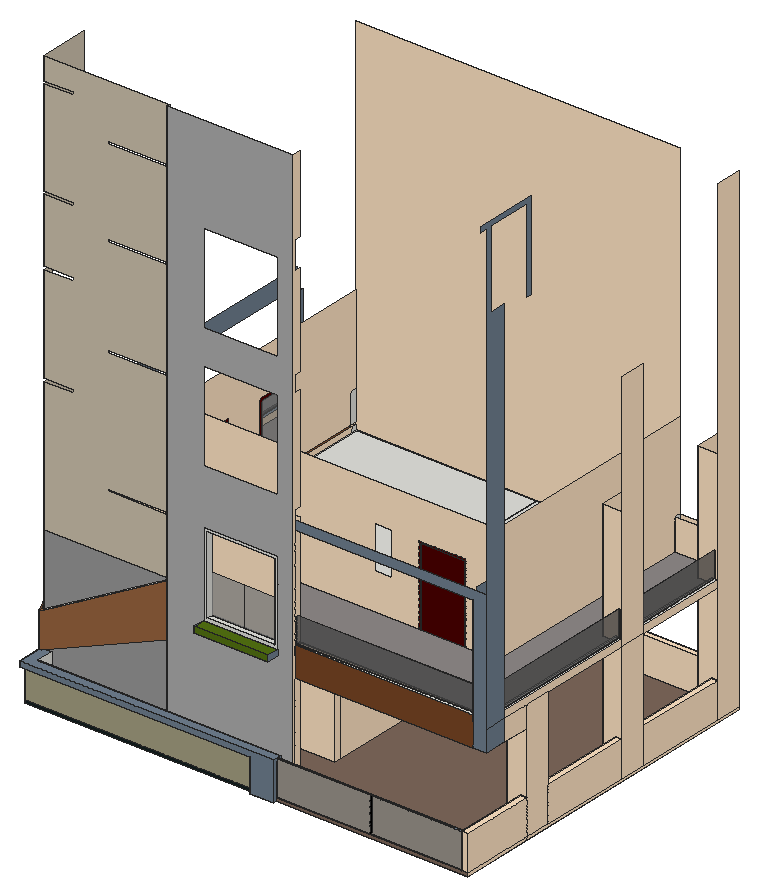
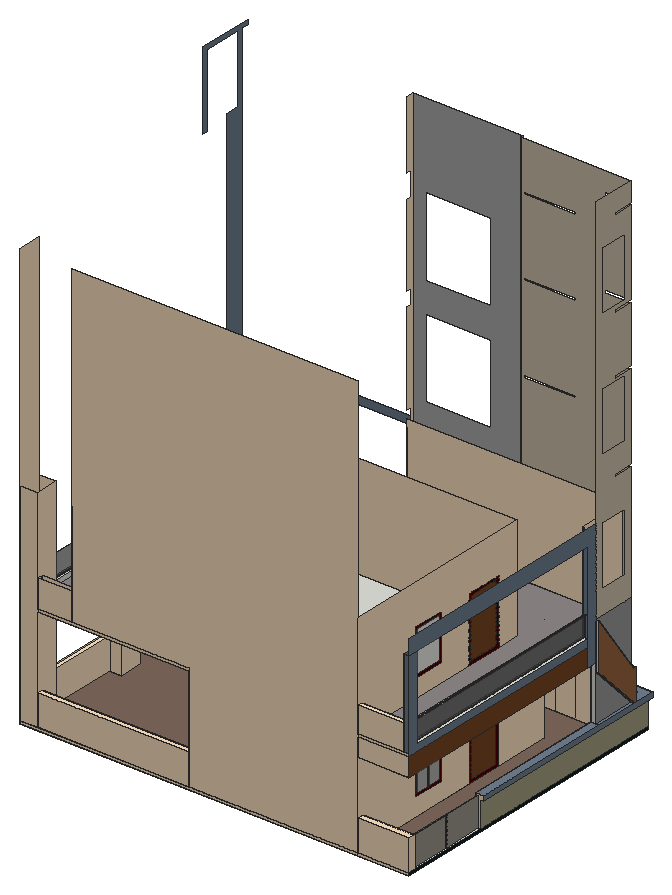
# SketchUp Ruby script. Lengths in inches.
U = 1.inch
M = Sketchup.active_model
def pt(a) = Geom::Point3d.new(a.map { |v| v * U })
def face(e, loops, mat)
  f = e.add_face(loops[0].map { |a| pt(a) })
  loops[1..].each { |l| e.add_face(l.map { |a| pt(a) }).erase! }
  f.material = f.back_material = mat if mat
  f
end
# faces: each face lists its corners as indices into pts; further lists are holes
def faces(e, pts, list, mat = nil) = list.each { |f| face(e, (f[0].is_a?(Array) ? f : [f]).map { |l| l.map { |i| pts[i] } }, mat) }
# xy, xz, yz: faces in a plane at the given z, y or x. An outline is a flat list of corners, or four numbers for a rectangle; further outlines are holes
def ring(l) = l.size == 4 ? [[l[0], l[1]], [l[2], l[1]], [l[2], l[3]], [l[0], l[3]]] : l.each_slice(2).to_a
def flat(e, list, mat, &to3) = list.each { |f| face(e, (f[0].is_a?(Array) ? f : [f]).map { |l| ring(l).map { |u, v| to3.(u, v) } }, mat) }
def xy(e, z, list, mat = nil) = flat(e, list, mat) { |x, y| [x, y, z] }
def xz(e, y, list, mat = nil) = flat(e, list, mat) { |x, z| [x, y, z] }
def yz(e, x, list, mat = nil) = flat(e, list, mat) { |y, z| [x, y, z] }
def lines(e, pts, list) = list.each { |a, b| e.add_line(pt(pts[a]), pt(pts[b])) }
# prism: a flat outline (further loops are holes) pulled along v
def prism(e, loops, v, mat = nil)
  f = face(e, loops, mat); d = Geom::Vector3d.new(v.map { |x| x * U })
  f.pushpull(f.normal.samedirection?(d) ? d.length : -d.length)
end
def box(e, o, s, mat = nil) = prism(e, [[o, [o[0] + s[0], o[1], o[2]], [o[0] + s[0], o[1] + s[1], o[2]], [o[0], o[1] + s[1], o[2]]]], [0, 0, s[2]], mat)
def at(x, y, z, deg = 0) = Geom::Transformation.translation(pt([x, y, z])) * Geom::Transformation.rotation(ORIGIN, Z_AXIS, deg.degrees)
def axes(o, x, y, z) = Geom::Transformation.new([*x, 0, *y, 0, *z, 0, *pt(o).to_a, 1])
def part(name) = M.definitions.add(name)
# library, detail: a bought-in or finely detailed component or shape, given as its bounding box
def library(name, o, s) = part(name).tap { |d| box(d.entities, o, s) }
def detail(e, o, s) = box(e.add_group.entities, o, s)
def put(e, d, t, mat = nil) = e.add_instance(d, t).tap { |i| i.material = mat if mat }
def group(e, t, mat = nil) = e.add_group.tap { |g| g.transformation = t; g.material = mat if mat }.entities
root = M.entities
M.materials.add("[0008_LavenderBlush]").color = [255, 240, 245]
M.materials.add("[0012_Bisque]").color = [255, 228, 196]
M.materials.add("[0021_DarkRed]").color = [76, 0, 0]
M.materials.add("[0021_DarkRed]1").color = [81, 0, 0]
M.materials.add("[0078_DarkSlateGray]").color = [19, 33, 33]
M.materials.add("[0111_SlateGray]").color = [112, 128, 144]
M.materials.add("[0136_Charcoal]").color = [35, 35, 35]
M.materials.add("[0137_Black]").color = [0, 0, 0]
M.materials.add("[Beadboard]").color = [153, 100, 63]
M.materials.add("[Carrera Marble]").color = [153, 153, 153]
M.materials.add("[Cladding Siding White]").color = [173, 173, 173]
M.materials.add("[Granite Brown]").color = [126, 104, 91]
M.materials.add("[Siding Rusty Metal]").color = [206, 195, 174]
M.materials.add("[Stone Coursed Rough]").color = [165, 160, 130]
M.materials.add("[Stone Marble]").color = [143, 138, 136]
M.materials.add("[Stone Masonry Multi]").color = [155, 149, 140]
M.materials.add("[Translucent Glass Gray]").color = [84, 84, 84]
M.materials["[Translucent Glass Gray]"].alpha = 0.5
M.materials.add("[Translucent Glass Gray]1").color = [128, 128, 128]
M.materials["[Translucent Glass Gray]1"].alpha = 0.5
M.materials.add("[Translucent Resin Crush Gray]").color = [153, 153, 153]
M.materials["[Translucent Resin Crush Gray]"].alpha = 0.8
M.materials.add("[Vegetation Blur 03]").color = [83, 114, 18]
M.materials.add("[Wood Veneer 01]").color = [120, 70, 37]
xy(root,0,[[948,0,948,12,24,12,24,1392,1824,1392,1824,12,1044,12,1044,0]])
xy(root,12,[[1044,12,1800,19.07],[1800,12,1824,312],[1044,19.07,1800,28.21],[1044,28.21,1800,36],[534,96,1044,108],
  [24,108,1044,132],[24,132,48,312],[24,312,48,978],[264,312,264,1392,1044,1392,1044,1368,288,1368,288,336,1044,336,1044,312],[1745,312,1824,420],
  [288,336,1020,1368],[1020,336,1044,1368],[1800,420,1824,798],[1745,798,1824,906],[1800,906,1824,1284],
  [24,978,36,1362],[36,978,41.76,1362],[41.76,978,48,1362],[1745,1284,1824,1392],[24,1362,264,1392],
  [1044,1368,1745,1392]])
xy(root,12,[[54,36,1800,36,1800,312,1745,312,1745,420,1800,420,1800,798,1745,798,1745,906,1800,906,1800,1284,1745,1284,1745,1368,1044,1368,1044,312,264,312,264,1362,48,1362,48,132,1044,132,1044,96,534,96,534,108,54,108]],"[Granite Brown]")
xy(root,19,[[1032,778.41,1044,981.6]],"[Wood Veneer 01]")
xy(root,132,[[12,0,12,978,24,978,24,12,948,12,948,0]],"[0111_SlateGray]")
xy(root,142.6875,[[1032,490.33,1044,626.21],[1032,1100.27,1044,1236.15]],"[Wood Veneer 01]")
xy(root,144.9375,[[36,978,41.76,1362]],"[Stone Masonry Multi]")
xy(root,151.1875,[[1044,19.07,1800,28.21]],"[0111_SlateGray]")
xy(root,156,[[1800,12,1824,312],[1800,420,1824,798],[1800,906,1824,1284],[24,1362,264,1392],[1044,1368,1745,1392]],"[0012_Bisque]")
xy(root,156,[[12,0,1044,0,1044,36,54,36,54,108,24,108,24,96,12,96],[12,108,24,312],[12,312,48,978]],"[0111_SlateGray]")
xy(root,156,[[12,96,24,108]],"[Beadboard]")
xy(root,300,[[12,96,24,108]],"[Beadboard]")
xy(root,335.4375,[[1032,490.33,1044,626.21],[1032,778.41,1044,981.6],[1032,1100.27,1044,1236.15]],"[Wood Veneer 01]")
xy(root,408,[[1800,132,1824,312]],"[0012_Bisque]")
xy(root,408,[[1044,108,1824,132],[24,312,24,1392,264,1392,264,1374,42,1374,42,312]],"[Wood Veneer 01]")
xy(root,471.68,[[683.08,48,983.45,96]],"[0111_SlateGray]")
xy(root,492,[[1800,132,1824,312],[288,336,1020,1368],[1020,336,1044,1368]])
xy(root,492,[[1298.29,369.5625,1292.07,370.38,1286.29,372.78,1281.32,376.59,1277.5,381.5625,1275.1,387.35,1274.29,393.5625,1275.1,399.77,1277.5,405.5625,1281.32,410.53,1286.29,414.35,1292.07,416.74,1298.29,417.5625,1304.5,416.74,1310.29,414.35,1315.26,410.53,1319.07,405.5625,1321.47,399.77,1322.29,393.5625,1321.47,387.35,1319.07,381.5625,1315.26,376.59,1310.29,372.78,1304.5,370.38],[1588.47,369.5625,1582.26,370.38,1576.47,372.78,1571.5,376.59,1567.6875,381.5625,1565.29,387.35,1564.47,393.5625,1565.29,399.77,1567.6875,405.5625,1571.5,410.53,1576.47,414.35,1582.26,416.74,1588.47,417.5625,1594.69,416.74,1600.47,414.35,1605.44,410.53,1609.26,405.5625,1611.66,399.77,1612.47,393.5625,1611.66,387.35,1609.26,381.5625,1605.44,376.59,1600.47,372.78,1594.69,370.38],[1588.47,625.0625,1582.26,625.88,1576.47,628.28,1571.5,632.09,1567.6875,637.0625,1565.29,642.85,1564.47,649.0625,1565.29,655.27,1567.6875,661.0625,1571.5,666.03,1576.47,669.85,1582.26,672.24,1588.47,673.0625,1594.69,672.24,1600.47,669.85,1605.44,666.03,1609.26,661.0625,1611.66,655.27,1612.47,649.0625,1611.66,642.85,1609.26,637.0625,1605.44,632.09,1600.47,628.28,1594.69,625.88],[1298.29,648.9375,1292.07,649.76,1286.29,652.15,1281.32,655.97,1277.5,660.9375,1275.1,666.73,1274.29,672.9375,1275.1,679.15,1277.5,684.9375,1281.32,689.91,1286.29,693.72,1292.07,696.12,1298.29,696.9375,1304.5,696.12,1310.29,693.72,1315.26,689.91,1319.07,684.9375,1321.47,679.15,1322.29,672.9375,1321.47,666.73,1319.07,660.9375,1315.26,655.97,1310.29,652.15,1304.5,649.76],[1588.47,1073.625,1582.26,1074.44,1576.47,1076.84,1571.5,1080.65,1567.6875,1085.625,1565.29,1091.41,1564.47,1097.625,1565.29,1103.84,1567.6875,1109.625,1571.5,1114.6,1576.47,1118.41,1582.26,1120.81,1588.47,1121.625,1594.69,1120.81,1600.47,1118.41,1605.44,1114.6,1609.26,1109.625,1611.66,1103.84,1612.47,1097.625,1611.66,1091.41,1609.26,1085.625,1605.44,1080.65,1600.47,1076.84,1594.69,1074.44],
  [1298.29,1135.0625,1292.07,1135.88,1286.29,1138.28,1281.32,1142.09,1277.5,1147.0625,1275.1,1152.85,1274.29,1159.0625,1275.1,1165.27,1277.5,1171.0625,1281.32,1176.03,1286.29,1179.85,1292.07,1182.24,1298.29,1183.0625,1304.5,1182.24,1310.29,1179.85,1315.26,1176.03,1319.07,1171.0625,1321.47,1165.27,1322.29,1159.0625,1321.47,1152.85,1319.07,1147.0625,1315.26,1142.09,1310.29,1138.28,1304.5,1135.88]],"[0008_LavenderBlush]")
xy(root,492,[[[48,132,48,312,1044,312,1044,1392,1745,1392,1745,1284,1824,1284,1824,906,1745,906,1745,798,1824,798,1824,420,1745,420,1745,312,1800,312,1800,132],[1588.47,1073.625,1594.69,1074.44,1600.47,1076.84,1605.44,1080.65,1609.26,1085.625,1611.66,1091.41,1612.47,1097.625,1611.66,1103.84,1609.26,1109.625,1605.44,1114.6,1600.47,1118.41,1594.69,1120.81,1588.47,1121.625,1582.26,1120.81,1576.47,1118.41,1571.5,1114.6,1567.6875,1109.625,1565.29,1103.84,1564.47,1097.625,1565.29,1091.41,1567.6875,1085.625,1571.5,1080.65,1576.47,1076.84,1582.26,1074.44],[1588.47,625.0625,1594.69,625.88,1600.47,628.28,1605.44,632.09,1609.26,637.0625,1611.66,642.85,1612.47,649.0625,1611.66,655.27,1609.26,661.0625,1605.44,666.03,1600.47,669.85,1594.69,672.24,1588.47,673.0625,1582.26,672.24,1576.47,669.85,1571.5,666.03,1567.6875,661.0625,1565.29,655.27,1564.47,649.0625,1565.29,642.85,1567.6875,637.0625,1571.5,632.09,1576.47,628.28,1582.26,625.88],[1588.47,369.5625,1594.69,370.38,1600.47,372.78,1605.44,376.59,1609.26,381.5625,1611.66,387.35,1612.47,393.5625,1611.66,399.77,1609.26,405.5625,1605.44,410.53,1600.47,414.35,1594.69,416.74,1588.47,417.5625,1582.26,416.74,1576.47,414.35,1571.5,410.53,1567.6875,405.5625,1565.29,399.77,1564.47,393.5625,1565.29,387.35,1567.6875,381.5625,1571.5,376.59,1576.47,372.78,1582.26,370.38],[1298.29,369.5625,1304.5,370.38,1310.29,372.78,1315.26,376.59,1319.07,381.5625,1321.47,387.35,1322.29,393.5625,1321.47,399.77,1319.07,405.5625,1315.26,410.53,1310.29,414.35,1304.5,416.74,1298.29,417.5625,1292.07,416.74,1286.29,414.35,1281.32,410.53,1277.5,405.5625,1275.1,399.77,1274.29,393.5625,1275.1,387.35,1277.5,381.5625,1281.32,376.59,1286.29,372.78,1292.07,370.38],[1298.29,648.9375,1304.5,649.76,1310.29,652.15,1315.26,655.97,1319.07,660.9375,1321.47,666.73,1322.29,672.9375,1321.47,679.15,1319.07,684.9375,1315.26,689.91,1310.29,693.72,1304.5,696.12,1298.29,696.9375,1292.07,696.12,1286.29,693.72,1281.32,689.91,1277.5,684.9375,1275.1,679.15,1274.29,672.9375,1275.1,666.73,1277.5,660.9375,1281.32,655.97,1286.29,652.15,1292.07,649.76],[1298.29,1135.0625,1304.5,1135.88,1310.29,1138.28,1315.26,1142.09,1319.07,1147.0625,1321.47,1152.85,1322.29,1159.0625,1321.47,1165.27,1319.07,1171.0625,1315.26,1176.03,1310.29,1179.85,1304.5,1182.24,1298.29,1183.0625,1292.07,1182.24,1286.29,1179.85,1281.32,1176.03,1277.5,1171.0625,1275.1,1165.27,1274.29,1159.0625,1275.1,1152.85,1277.5,1147.0625,1281.32,1142.09,1286.29,1138.28,1292.07,1135.88]],[42,312,264,1374]],"[Wood Veneer 01]")
xy(root,495.68,[[683.08,48,983.45,96]],"[Vegetation Blur 03]")
xy(root,504,[[48,1368,264,1392],[1584,1368,1745,1392]])
xy(root,504,[[48,132,1767.4375,132,1767.4375,199.52,1800,199.52,1800,798,1745,798,1745,906,1800,906,1800,1284,1745,1284,1745,1368,1584,1368,1584,468,1446.53,468,1446.53,469.5,1268.41,469.5,1268.41,468,264,468,264,1368,48,1368]],"[Stone Marble]")
xy(root,507.68,[[695.08,96,971.45,120]])
xy(root,522,[[1800,199.52,1812,798],[1812,199.52,1813.5,798],[1813.5,199.52,1824,798],[1800,906,1812,1284],[1812,906,1813.5,1284],
  [1813.5,906,1824,1284]])
xy(root,528,[[1044,108,1767.4375,118.5],[1044,118.5,1767.4375,120],[24,360,35,1350],[35,360,36,1350]])
xy(root,528,[[1044,120,1767.4375,132]],"[0012_Bisque]")
xy(root,528,[[36,360,48,1350]],"[0111_SlateGray]")
xy(root,621,[[35,360,36,1350]])
xy(root,624,[[48,1368,264,1392]],"[0012_Bisque]")
xz(root,0,[[948,0,1044,0,1044,156,12,156,12,132,948,132]],"[0111_SlateGray]")
xz(root,12,[[1800,12,1824,156]],"[0012_Bisque]")
xz(root,12,[[24,0,948,12]],"[0078_DarkSlateGray]")
xz(root,12,[[1044,0,1824,12]],"[Granite Brown]")
xz(root,12,[[24,12,948,132]],"[Stone Coursed Rough]")
xz(root,19.07,[[1422,12,1429.54,151.1875]],"[0137_Black]")
xz(root,19.07,[[1044,12,1422,151.1875],[1429.54,12,1800,151.1875]],"[Stone Masonry Multi]")
xz(root,28.21,[[1044,12,1800,151.1875]],"[Stone Masonry Multi]")
xz(root,36,[[54,12,1044,156]])
xz(root,48,[[683.08,471.68,983.45,495.68]],"[Vegetation Blur 03]")
xz(root,96,[[683.08,471.68,983.45,495.68],[[683.08,495.68,983.45,837.43],[695.08,507.68,971.45,825.43]]])
xz(root,96,[[12,156,24,156,534,373.64,534,588,24,300,12,300]],"[Beadboard]")
xz(root,96,[[[534,12,1044,2319.6],[683.08,471.68,983.45,837.43],[683.08,1057.8,983.45,1423.55],[683.08,1562.74,983.45,1928.49]]],"[Cladding Siding White]")
xz(root,108,[[24,156,24,300,534,588,534,373.64]])
xz(root,108,[[1767.4375,408,1824,408,1824,984,1044,984,1044,948,1767.4375,948]],"[0111_SlateGray]")
xz(root,108,[[54,12,534,12,534,373.64,24,156,54,156],[24,300,534,588,24,588]],"[Carrera Marble]")
xz(root,108,[[[24,588,534,588,534,2319.6,24,2319.6,24,2228.39,144,2228.39,144,2216.39,24,2216.39,24,1825.2,144,1825.2,144,1813.2,24,1813.2,24,1551.33,144,1551.33,144,1539.33,24,1539.33,24,1142.7,144,1142.7,144,1130.7,24,1130.7],[282.03,2087.13,522.41,2097.5],[282.03,1731.25,522.41,1741.63],[282.03,1326.13,522.41,1336.5],[282.03,820.69,522.41,831.07]]],"[Siding Rusty Metal]")
xz(root,108,[[1044,408,1767.4375,528]],"[Wood Veneer 01]")
xz(root,118.5,[[1044,528,1767.4375,633]],"[Translucent Glass Gray]")
xz(root,120,[[1044,528,1767.4375,633]],"[Translucent Glass Gray]")
xz(root,120,[[695.08,507.68,833.27,666.55],[833.27,507.68,971.45,666.55]],"[Translucent Resin Crush Gray]")
xz(root,132,[[264,492,358.73,504],[358.73,492,1044,504]])
xz(root,132,[[48,12,264,492],[264,12,358.73,492],[358.73,12,358.73,492,1800,492,1800,408,1044,408,1044,12],[48,504,1044,984],[1044,504,1767.4375,528]],"[0012_Bisque]")
xz(root,199.52,[[1800,504,1824,522],[1812,522,1813.5,627]])
xz(root,199.52,[[[1767.4375,504,1767.4375,984,1824,984,1824,522,1800,522,1800,504],[1812,627,1812.78,627.1,1813.5,627.4,1814.12,627.88,1814.6,628.5,1814.9,629.22,1815,630,1814.9,630.78,1814.6,631.5,1814.12,632.12,1813.5,632.6,1812.78,632.9,1812,633,1811.22,632.9,1810.5,632.6,1809.88,632.12,1809.4,631.5,1809.1,630.78,1809,630,1809.1,629.22,1809.4,628.5,1809.88,627.88,1810.5,627.4,1811.22,627.1]]],"[0111_SlateGray]")
xz(root,312,[[1800,12,1824,156],[24,156,24,408,42,408,42,492,48,492,48,156],[12,373.64,24,588],[24,408,42,492],[1800,408,1824,492]])
xz(root,312,[[264,12,1044,492],[1745,12,1800,12,1800,156,1824,156,1824,408,1800,408,1800,492,1745,492]],"[0012_Bisque]")
xz(root,336,[[288,12,1020,492],[1020,12,1044,492]])
xz(root,360,[[35,528,36,621]])
xz(root,360,[[[24,528,24,912,42,912,42,984,48,984,48,528],[36,621,36.78,621.1,37.5,621.4,38.12,621.88,38.6,622.5,38.9,623.22,39,624,38.9,624.78,38.6,625.5,38.12,626.12,37.5,626.6,36.78,626.9,36,627,35.22,626.9,34.5,626.6,33.88,626.12,33.4,625.5,33.1,624.78,33,624,33.1,623.22,33.4,622.5,33.88,621.88,34.5,621.4,35.22,621.1]]],"[0111_SlateGray]")
xz(root,420,[[1745,12,1745,492,1824,492,1824,156,1800,156,1800,12],[1800,12,1824,156]])
xz(root,468,[[[264,504,1260.41,504,1260.41,827.1875,1454.53,827.1875,1454.53,504,1584,504,1584,984,264,984],[1080.18,652.0625,1153.12,827.1875]]],"[0012_Bisque]")
xz(root,468,[[1260.41,504,1268.41,504,1268.41,819.1875,1446.53,819.1875,1446.53,504,1454.53,504,1454.53,827.1875,1260.41,827.1875]],"[0021_DarkRed]")
xz(root,469.5,[[1268.41,504,1446.53,819.1875]],"[0021_DarkRed]")
xz(root,490.33,[[1032,142.6875,1044,335.4375]],"[Wood Veneer 01]")
xz(root,626.21,[[1032,142.6875,1044,335.4375]],"[Wood Veneer 01]")
xz(root,778.41,[[1032,19,1044,335.4375]],"[Wood Veneer 01]")
xz(root,798,[[1800,12,1824,156],[1800,504,1824,522],[1812,522,1813.5,627]])
xz(root,798,[[1745,12,1800,12,1800,156,1824,156,1824,492,1745,492],[[1745,504,1800,504,1800,522,1824,522,1824,984,1745,984],[1812,627,1811.22,627.1,1810.5,627.4,1809.88,627.88,1809.4,628.5,1809.1,629.22,1809,630,1809.1,630.78,1809.4,631.5,1809.88,632.12,1810.5,632.6,1811.22,632.9,1812,633,1812.78,632.9,1813.5,632.6,1814.12,632.12,1814.6,631.5,1814.9,630.78,1815,630,1814.9,629.22,1814.6,628.5,1814.12,627.88,1813.5,627.4,1812.78,627.1]]],"[0012_Bisque]")
xz(root,906,[[1800,12,1824,156],[1800,504,1824,522],[1812,522,1813.5,627]])
xz(root,906,[[1745,12,1745,492,1824,492,1824,156,1800,156,1800,12],[[1745,504,1745,984,1824,984,1824,522,1800,522,1800,504],[1812,627,1812.78,627.1,1813.5,627.4,1814.12,627.88,1814.6,628.5,1814.9,629.22,1815,630,1814.9,630.78,1814.6,631.5,1814.12,632.12,1813.5,632.6,1812.78,632.9,1812,633,1811.22,632.9,1810.5,632.6,1809.88,632.12,1809.4,631.5,1809.1,630.78,1809,630,1809.1,629.22,1809.4,628.5,1809.88,627.88,1810.5,627.4,1811.22,627.1]]],"[0012_Bisque]")
xz(root,978,[[36,12,41.76,144.9375]])
xz(root,978,[[24,12,24,132,12,132,12,156,48,156,48,12,41.76,12,41.76,144.9375,36,144.9375,36,12]],"[0012_Bisque]")
xz(root,981.6,[[1032,19,1044,335.4375]],"[Wood Veneer 01]")
xz(root,1100.27,[[1032,142.6875,1044,335.4375]],"[Wood Veneer 01]")
xz(root,1236.15,[[1032,142.6875,1044,335.4375]],"[Wood Veneer 01]")
xz(root,1284,[[1800,12,1824,156],[1800,504,1824,522],[1812,522,1813.5,627]])
xz(root,1284,[[1745,12,1800,12,1800,156,1824,156,1824,492,1745,492],[[1745,504,1800,504,1800,522,1824,522,1824,984,1745,984],[1812,627,1811.22,627.1,1810.5,627.4,1809.88,627.88,1809.4,628.5,1809.1,629.22,1809,630,1809.1,630.78,1809.4,631.5,1809.88,632.12,1810.5,632.6,1811.22,632.9,1812,633,1812.78,632.9,1813.5,632.6,1814.12,632.12,1814.6,631.5,1814.9,630.78,1815,630,1814.9,629.22,1814.6,628.5,1814.12,627.88,1813.5,627.4,1812.78,627.1]]],"[0012_Bisque]")
xz(root,1350,[[35,528,36,621],[36,621,35.22,621.1,34.5,621.4,33.88,621.88,33.4,622.5,33.1,623.22,33,624,33.1,624.78,33.4,625.5,33.88,626.12,34.5,626.6,35.22,626.9,36,627,36.78,626.9,37.5,626.6,38.12,626.12,38.6,625.5,38.9,624.78,39,624,38.9,623.22,38.6,622.5,38.12,621.88,37.5,621.4,36.78,621.1]])
xz(root,1350,[[[24,528,48,912],[36,621,35.22,621.1,34.5,621.4,33.88,621.88,33.4,622.5,33.1,623.22,33,624,33.1,624.78,33.4,625.5,33.88,626.12,34.5,626.6,35.22,626.9,36,627,36.78,626.9,37.5,626.6,38.12,626.12,38.6,625.5,38.9,624.78,39,624,38.9,623.22,38.6,622.5,38.12,621.88,37.5,621.4,36.78,621.1]]],"[0111_SlateGray]")
xz(root,1362,[[36,12,41.76,144.9375]])
xz(root,1362,[[24,12,36,12,36,144.9375,41.76,144.9375,41.76,12,48,12,48,156,24,156],[48,12,264,156]],"[0012_Bisque]")
xz(root,1368,[[288,12,1020,492],[1020,12,1044,492]])
xz(root,1368,[[1044,12,1745,156],[48,504,264,624],[1584,504,1745,632.12]],"[0012_Bisque]")
xz(root,1374,[[42,408,264,492]],"[Wood Veneer 01]")
xz(root,1392,[[24,0,264,12],[264,0,1824,12],[24,12,264,156],[264,12,264,1968,1584,1968,1584,504,1044,504,1044,12],[1044,12,1745,156],
  [1745,12,1824,984],[24,408,264,492],[24,492,264,504],[1044,492,1745,504],[48,504,264,624],
  [1584,504,1745,632.12]],"[0012_Bisque]")
xz(root,1392,[[24,504,48,912]],"[0111_SlateGray]")
yz(root,12,[[0,132,978,156]],"[0111_SlateGray]")
yz(root,12,[[96,156,96,300,108,300,312,588,312,373.64,108,156]],"[Beadboard]")
yz(root,24,[[108,156,312,373.64,312,588,108,300]])
yz(root,24,[[1362,12,1392,156]],"[0012_Bisque]")
yz(root,24,[[12,0,1392,12]],"[0078_DarkSlateGray]")
yz(root,24,[[312,408,312,984,1392,984,1392,912,360,912,360,408],[360,492,360,528,1350,528,1350,912,1392,912,1392,492]],"[0111_SlateGray]")
yz(root,24,[[108,156,312,373.64,312,156],[108,300,108,588,312,588]],"[Carrera Marble]")
yz(root,24,[[[108,588,108,1130.7,204,1130.7,204,1142.7,108,1142.7,108,1539.33,204,1539.33,204,1551.33,108,1551.33,108,1813.2,204,1813.2,204,1825.2,108,1825.2,108,2216.39,204,2216.39,204,2228.39,108,2228.39,108,2319.6,312,2319.6,312,588],[146.55,700.8125,276.68,974.8125],[146.55,1256.625,276.68,1530.625],[146.55,1839.3125,276.68,2113.3125]]],"[Siding Rusty Metal]")
yz(root,24,[[12,12,978,132]],"[Stone Coursed Rough]")
yz(root,24,[[360,408,1392,492]],"[Wood Veneer 01]")
yz(root,35,[[360,528,1350,621]],"[Translucent Glass Gray]")
yz(root,36,[[360,621,1350,624]])
yz(root,36,[[1159.83,12,1170,144.9375]],"[0136_Charcoal]")
yz(root,36,[[978,12,1159.83,144.9375],[1170,12,1362,144.9375]],"[Stone Masonry Multi]")
yz(root,36,[[360,528,1350,621]],"[Translucent Glass Gray]")
yz(root,41.76,[[978,12,1362,144.9375]],"[Stone Masonry Multi]")
yz(root,42,[[312,408,1374,492]],"[Wood Veneer 01]")
yz(root,48,[[1368,504,1392,528],[1350,528,1368,624],[1368,528,1392,624]])
yz(root,48,[[132,12,312,492],[312,12,978,156],[132,504,1368,504,1368,528,360,528,360,984,132,984]],"[0012_Bisque]")
yz(root,48,[[1350,624,1392,912]],"[0111_SlateGray]")
yz(root,54,[[36,12,108,156]])
yz(root,264,[[1362,12,1392,156],[1374,408,1392,492],[1368,504,1392,624]])
yz(root,264,[[[312,12,312,492,1374,492,1374,408,1392,408,1392,156,1362,156,1362,12,745.46,12,745.46,286.3125,575.92,286.3125,575.92,12],[904.02,91.5,1059.83,286.3125]],[[468,504,468,984,1392,984,1392,624,1368,624,1368,504,745.46,504,745.46,801.1,575.92,801.1,575.92,504],[904.02,584.5,1060.8,801.1]]],"[0012_Bisque]")
yz(root,264,[[[575.92,12,745.46,286.3125],[587.92,24,733.46,274.3125]],[[904.02,91.5,1059.83,286.3125],[916.02,103.5,1047.83,274.3125]],[976.93,103.5,986.93,274.3125],[[575.92,504,745.46,801.1],[587.92,516,733.46,789.1]],[[904.02,584.5,1060.8,801.1],[916.02,596.5,1048.8,789.1]]],"[0021_DarkRed]1")
yz(root,264,[[916.02,103.5,976.93,274.3125],[986.93,103.5,1047.83,274.3125],[916.02,596.5,1048.8,789.1]],"[Translucent Glass Gray]1")
yz(root,264,[[587.92,24,733.46,274.3125],[587.92,516,733.46,789.1]],"[Wood Veneer 01]")
yz(root,288,[[336,12,1368,468],[336,468,1368,492]])
yz(root,534,[[96,373.64,108,588]])
yz(root,534,[[96,12,108,373.64]],"[Carrera Marble]")
yz(root,534,[[96,588,108,2319.6]],"[Cladding Siding White]")
yz(root,683.08,[[48,471.68,96,495.68]],"[0111_SlateGray]")
yz(root,695.08,[[96,507.68,120,825.43]])
yz(root,948,[[0,0,12,132]],"[0111_SlateGray]")
yz(root,971.45,[[96,507.68,120,825.43]])
yz(root,983.45,[[48,471.68,96,495.68]],"[0111_SlateGray]")
yz(root,1020,[[336,12,1368,492]])
yz(root,1032,[[490.33,142.6875,626.21,335.4375],[1100.27,142.6875,1236.15,335.4375]])
yz(root,1032,[[778.41,19,981.6,335.4375]],"[Wood Veneer 01]")
yz(root,1044,[[19.07,12,28.21,151.1875],[1368,12,1392,156],[108,492,132,504],[108,504,132,528],[118.5,528,120,633]])
yz(root,1044,[[[96,12,108,12,108,1020,132,1020,132,1446,108,1446,108,1512,132,1512,132,1891.5,108,1891.5,108,2004,132,2004,132,2319.6,96,2319.6],[120,2103,119.6875,2103.02,119.375,2103.07,119.07,2103.15,118.78,2103.26,118.5,2103.4,118.24,2103.57,117.99,2103.77,117.77,2103.99,117.57,2104.24,117.4,2104.5,117.26,2104.78,117.15,2105.07,117.07,2105.375,117.02,2105.6875,117,2106,117.02,2106.3125,117.07,2106.625,117.15,2106.93,117.26,2107.22,117.4,2107.5,117.57,2107.76,117.77,2108.01,117.99,2108.23,118.24,2108.43,118.5,2108.6,118.78,2108.74,119.07,2108.85,119.375,2108.93,119.6875,2108.98,120,2109,120.3125,2108.98,120.625,2108.93,120.93,2108.85,121.22,2108.74,121.5,2108.6,121.76,2108.43,122.01,2108.23,122.23,2108.01,122.43,2107.76,122.6,2107.5,122.74,2107.22,122.85,2106.93,122.93,2106.625,122.98,2106.3125,123,2106,122.98,2105.6875,122.93,2105.375,122.85,2105.07,122.74,2104.78,122.6,2104.5,122.43,2104.24,122.23,2103.99,122.01,2103.77,121.76,2103.57,121.5,2103.4,121.22,2103.26,120.93,2103.15,120.625,2103.07,120.3125,2103.02],[120,1125.02,119.53,1125.04,118.78,1125.26,118.5,1125.43,118.11,1125.67,117.57,1126.24,117.2,1126.92,117.02,1127.6875,117.04,1128.47,117.26,1129.22,117.67,1129.89,118.24,1130.43,118.92,1130.8,119.6875,1130.98,120.47,1130.96,121.22,1130.74,121.89,1130.33,122.43,1129.76,122.8,1129.08,122.98,1128.3125,122.96,1127.53,122.74,1126.78,122.33,1126.11,121.76,1125.57,121.08,1125.2,120.3125,1125.02],[120,1617,119.22,1617.1,118.5,1617.4,117.88,1617.88,117.4,1618.5,117.1,1619.22,117,1620,117.1,1620.78,117.4,1621.5,117.88,1622.12,118.5,1622.6,119.22,1622.9,120,1623,120.78,1622.9,121.5,1622.6,122.12,1622.12,122.6,1621.5,122.9,1620.78,123,1620,122.9,1619.22,122.6,1618.5,122.12,1617.88,121.5,1617.4,120.78,1617.1]],[108,12,132,408],[312,12,336,492],[[336,12,771.41,12,771.41,342.4375,988.6,342.4375,988.6,12,1368,12,1368,492,336,492],[1093.27,135.6875,1243.15,342.4375],[483.33,135.6875,633.21,342.4375]],[1368,156,1392,492],
  [[108,528,132,948],[120,633,119.22,633.1,118.5,633.4,117.88,633.88,117.4,634.5,117.1,635.22,117,636,117.1,636.78,117.4,637.5,117.88,638.12,118.5,638.6,119.22,638.9,120,639,120.78,638.9,121.5,638.6,122.12,638.12,122.6,637.5,122.9,636.78,123,636,122.9,635.22,122.6,634.5,122.12,633.88,121.5,633.4,120.78,633.1]]],"[0012_Bisque]")
yz(root,1044,[[0,0,12,0,12,12,19.07,12,19.07,151.1875,28.21,151.1875,28.21,12,36,12,36,156,0,156]],"[0111_SlateGray]")
yz(root,1044,[[[771.41,12,988.6,342.4375],[778.41,19,981.6,335.4375]],[[483.33,135.6875,633.21,342.4375],[490.33,142.6875,626.21,335.4375]],[[1093.27,135.6875,1243.15,342.4375],[1100.27,142.6875,1236.15,335.4375]]],"[Wood Veneer 01]")
yz(root,1268.41,[[468,504,469.5,819.1875]])
yz(root,1446.53,[[468,504,469.5,819.1875]])
yz(root,1584,[[1368,504,1392,632.12]])
yz(root,1584,[[468,504,1368,504,1368,632.12,1392,632.12,1392,984,468,984]],"[0012_Bisque]")
yz(root,1745,[[1368,12,1392,156],[1368,504,1392,632.12]])
yz(root,1745,[[312,12,420,492],[798,12,906,492],[1284,12,1284,492,1392,492,1392,156,1368,156,1368,12],[798,504,906,984],[1284,504,1284,984,1392,984,1392,632.12,1368,632.12,1368,504]],"[0012_Bisque]")
yz(root,1767.4375,[[108,504,132,528],[118.5,528,120,633]])
yz(root,1767.4375,[[[132,504,132,528,108,528,108,948,132,948,132,984,199.52,984,199.52,504],[120,633,120.78,633.1,121.5,633.4,122.12,633.88,122.6,634.5,122.9,635.22,123,636,122.9,636.78,122.6,637.5,122.12,638.12,121.5,638.6,120.78,638.9,120,639,119.22,638.9,118.5,638.6,117.88,638.12,117.4,637.5,117.1,636.78,117,636,117.1,635.22,117.4,634.5,117.88,633.88,118.5,633.4,119.22,633.1]]],"[0111_SlateGray]")
yz(root,1800,[[12,12,12,156,36,156,36,12,28.21,12,28.21,151.1875,19.07,151.1875,19.07,12],[19.07,12,28.21,151.1875],[199.52,504,798,522],[906,504,1284,522]])
yz(root,1800,[[36,12,312,156],[420,12,798,156],[906,12,1284,156],[132,408,312,492]],"[0012_Bisque]")
yz(root,1812,[[199.52,522,798,627],[906,522,1284,627]],"[Translucent Glass Gray]")
yz(root,1813.5,[[199.52,522,798,627],[906,522,1284,627]],"[Translucent Glass Gray]")
yz(root,1824,[[12,0,312,12],[312,0,1392,12],[12,12,312,156],[312,12,420,492],[420,12,798,156],
  [798,12,906,492],[906,12,1284,156],[1284,12,1392,1968],[199.52,408,312,492],[199.52,492,798,522],
  [798,492,906,1476],[906,492,1284,522]],"[0012_Bisque]")
yz(root,1824,[[108,408,199.52,492],[108,492,199.52,492,199.52,2004,132,2004,132,2319.6,312,2319.6,312,1980,336,1980,336,2340,78,2340,78,2319.6,108,2319.6]],"[0111_SlateGray]")
p = [[24,108,156],[534,108,373.64],[534,96,373.64],[24,96,156],[24,312,373.64],[12,108,156],
  [12,312,373.64],[534,108,588],[24,108,300],[24,96,300],[534,96,588],[24,312,588],
  [12,312,588],[12,108,300],[35.22,1350,621.1],[36,1350,621],[36,360,621],[35.22,360,621.1],
  [36.78,1350,621.1],[36.78,360,621.1],[34.5,1350,621.4],[34.5,360,621.4],[37.5,1350,621.4],[37.5,360,621.4],
  [33.88,1350,621.88],[33.88,360,621.88],[38.12,1350,621.88],[38.12,360,621.88],[33.4,1350,622.5],[33.4,360,622.5],
  [38.6,1350,622.5],[38.6,360,622.5],[33.1,1350,623.22],[33.1,360,623.22],[38.9,1350,623.22],[38.9,360,623.22],
  [33,1350,624],[33,360,624],[39,1350,624],[39,360,624],[33.1,1350,624.78],[33.1,360,624.78],
  [38.9,1350,624.78],[38.9,360,624.78],[33.4,1350,625.5],[33.4,360,625.5],[38.6,1350,625.5],[38.6,360,625.5],
  [33.88,1350,626.12],[33.88,360,626.12],[38.12,1350,626.12],[38.12,360,626.12],[264,312,0],[264,312,12],
  [264,312,492],[264,312,504],[24,312,504],[48,312,504],[24,312,528],[48,312,528]]
faces(root,p,[[0,1,2,3],[4,0,5,6],[7,8,9,10],[8,11,12,13]],"[Beadboard]")
faces(root,p,[[14,15,16,17],[15,18,19,16],[20,14,17,21],[18,22,23,19],[24,20,21,25],[22,26,27,23],[28,24,25,29],[26,30,31,27],
  [32,28,29,33],[30,34,35,31],[36,32,33,37],[34,38,39,35],[40,36,37,41],[38,42,43,39],[44,40,41,45],[42,46,47,43],
  [48,44,45,49],[46,50,51,47]])
lines(root,p,[[52,53],[54,55],[56,57],[58,59]])
